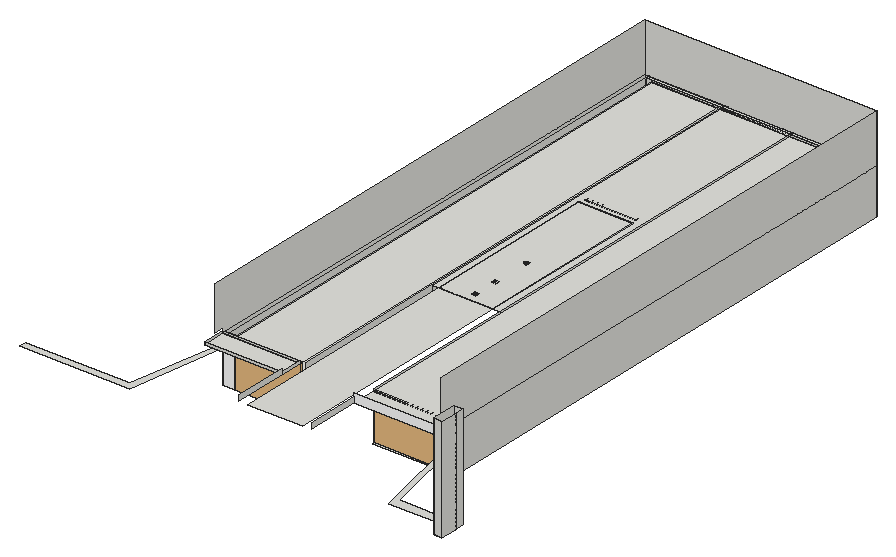
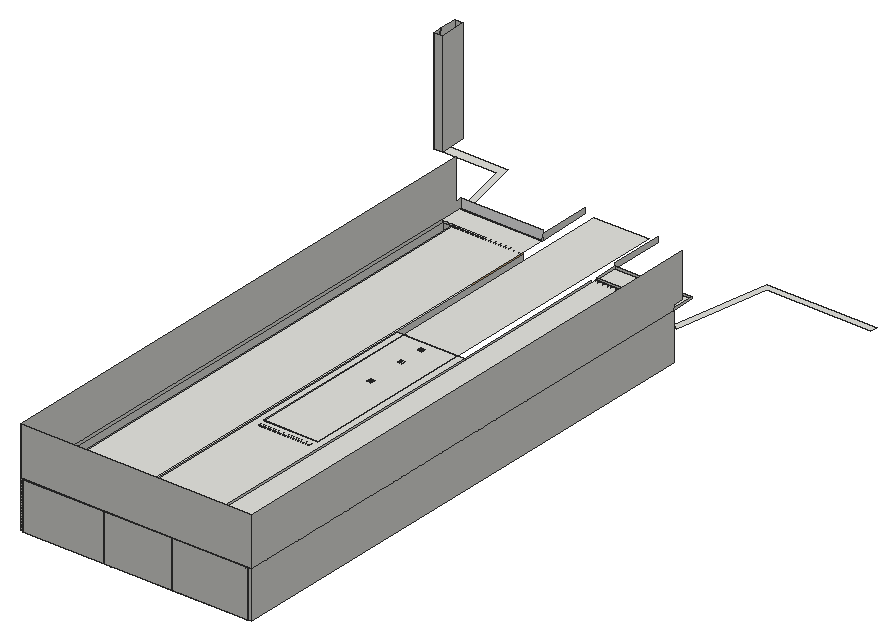
# SketchUp Ruby script. Lengths in inches.
U = 1.inch
M = Sketchup.active_model
def pt(a) = Geom::Point3d.new(a.map { |v| v * U })
def face(e, loops, mat)
  f = e.add_face(loops[0].map { |a| pt(a) })
  loops[1..].each { |l| e.add_face(l.map { |a| pt(a) }).erase! }
  f.material = f.back_material = mat if mat
  f
end
# faces: each face lists its corners as indices into pts; further lists are holes
def faces(e, pts, list, mat = nil) = list.each { |f| face(e, (f[0].is_a?(Array) ? f : [f]).map { |l| l.map { |i| pts[i] } }, mat) }
# xy, xz, yz: faces in a plane at the given z, y or x. An outline is a flat list of corners, or four numbers for a rectangle; further outlines are holes
def ring(l) = l.size == 4 ? [[l[0], l[1]], [l[2], l[1]], [l[2], l[3]], [l[0], l[3]]] : l.each_slice(2).to_a
def flat(e, list, mat, &to3) = list.each { |f| face(e, (f[0].is_a?(Array) ? f : [f]).map { |l| ring(l).map { |u, v| to3.(u, v) } }, mat) }
def xy(e, z, list, mat = nil) = flat(e, list, mat) { |x, y| [x, y, z] }
def xz(e, y, list, mat = nil) = flat(e, list, mat) { |x, z| [x, y, z] }
def yz(e, x, list, mat = nil) = flat(e, list, mat) { |y, z| [x, y, z] }
def lines(e, pts, list) = list.each { |a, b| e.add_line(pt(pts[a]), pt(pts[b])) }
# prism: a flat outline (further loops are holes) pulled along v
def prism(e, loops, v, mat = nil)
  f = face(e, loops, mat); d = Geom::Vector3d.new(v.map { |x| x * U })
  f.pushpull(f.normal.samedirection?(d) ? d.length : -d.length)
end
def box(e, o, s, mat = nil) = prism(e, [[o, [o[0] + s[0], o[1], o[2]], [o[0] + s[0], o[1] + s[1], o[2]], [o[0], o[1] + s[1], o[2]]]], [0, 0, s[2]], mat)
def at(x, y, z, deg = 0) = Geom::Transformation.translation(pt([x, y, z])) * Geom::Transformation.rotation(ORIGIN, Z_AXIS, deg.degrees)
def axes(o, x, y, z) = Geom::Transformation.new([*x, 0, *y, 0, *z, 0, *pt(o).to_a, 1])
def part(name) = M.definitions.add(name)
# library, detail: a bought-in or finely detailed component or shape, given as its bounding box
def library(name, o, s) = part(name).tap { |d| box(d.entities, o, s) }
def detail(e, o, s) = box(e.add_group.entities, o, s)
def put(e, d, t, mat = nil) = e.add_instance(d, t).tap { |i| i.material = mat if mat }
def group(e, t, mat = nil) = e.add_group.tap { |g| g.transformation = t; g.material = mat if mat }.entities
root = M.entities
M.materials.add("[Color M00]").color = [255, 255, 255]
c1 = library("Group\#4",[0,0,0],[146.0625,8.01,104.72])
c2 = library("Sliding Door",[0,0,0],[94.49,5.83,91.73])
c3 = library("Group5_1",[-7.56,-66.38,0.11],[6.33,135.04,120.95])
c4 = library("Omni Light\#4",[-12,-12,-12],[24,24,24])
c5 = library("Omni Light\#3",[-12,-12,-12],[24,24,24])
c6 = library("Spot Light",[-5.1,-5.1,-11.05],[10.2,10.2,11.05])
c7 = library("Spot Light\#1",[-5.1,-5.1,-11.05],[10.2,10.2,11.05])
c8 = library("Spot Light\#2",[-5.1,-5.1,-11.05],[10.2,10.2,11.05])
xy(root,34.97,[[765.09,749.51,934.66,2093.94],[1121.6,749.51,1301.45,2093.94],[744.92,758.51,765.09,758.51,765.09,2093.94,934.66,2093.94,934.66,976.22,940.98,976.22,940.98,2100.75,744.92,2100.75],[934.66,758.51,940.98,928.22],[1115.98,758.51,1121.6,758.51,1121.6,2093.94,1301.45,2093.94,1301.45,758.51,1323.45,758.51,1323.45,2100.75,1115.98,2100.75],
  [934.66,928.22,940.98,976.22],[940.98,2093.94,963.8,2100.75],[963.8,2093.94,1093.61,2100.75],[1093.61,2093.94,1115.98,2100.75],[744.92,2100.75,940.98,2109.75],
  [940.98,2100.75,963.8,2109.75],[963.8,2100.75,1093.61,2109.75],[1093.61,2100.75,1115.98,2109.75],[1115.98,2100.75,1323.45,2109.75],[744.92,2109.75,963.8,2111.5625],
  [963.8,2109.75,1093.61,2111.5625],[1093.61,2109.75,1323.45,2111.5625]])
xy(root,118.97,[[934.66,928.22,940.98,976.22],[940.98,928.22,958.48,976.22],[1098.48,937.55,1107.36,985.55]])
xy(root,120.65,[[1545.43,417,1548.46,459.625],[1548.46,417,1566.68,459.625],[1395.9,459.625,1545.43,459.625,1545.43,482.75,1404.4,482.75,1345.66,749.51,1332.45,749.51],[1545.43,459.625,1548.46,482.75],[1548.46,459.625,1566.68,463.0625],
  [1548.46,463.0625,1566.68,482.75],[411.47,500.87,693.04,500.87,735.92,749.51,721.7,754.86,678.72,519.18,411.47,519.18]])
xy(root,148.22,[[963.8,1617.7,1093.61,2109.75]])
xy(root,154.53,[[[958.48,1166.95,1098.48,1617.7],[1031.74,1351.9,1032.77,1352.04,1033.74,1352.4375,1034.57,1353.07,1035.2,1353.9,1035.6,1354.87,1035.74,1355.9,1035.6,1356.9375,1035.2,1357.9,1034.57,1358.73,1033.74,1359.37,1032.77,1359.76,1031.74,1359.9,1030.7,1359.76,1029.74,1359.37,1028.91,1358.73,1028.28,1357.9,1027.875,1356.9375,1027.74,1355.9,1027.875,1354.87,1028.28,1353.9,1028.91,1353.07,1029.74,1352.4375,1030.7,1352.04],[1031.74,1189.09,1032.77,1189.23,1033.74,1189.625,1034.57,1190.26,1035.2,1191.09,1035.6,1192.06,1035.74,1193.09,1035.6,1194.125,1035.2,1195.09,1034.57,1195.92,1033.74,1196.55,1032.77,1196.95,1031.74,1197.09,1030.7,1196.95,1029.74,1196.55,1028.91,1195.92,1028.28,1195.09,1027.875,1194.125,1027.74,1193.09,1027.875,1192.06,1028.28,1191.09,1028.91,1190.26,1029.74,1189.625,1030.7,1189.23],[1031.74,1254.99,1032.16,1255.05,1032.55,1255.21,1032.89,1255.47,1033.15,1255.81,1033.31,1256.2,1033.36,1256.62,1033.31,1257.04,1033.15,1257.43,1032.89,1257.77,1032.55,1258.03,1032.16,1258.1875,1031.74,1258.24,1031.32,1258.1875,1030.93,1258.03,1030.59,1257.77,1030.33,1257.43,1030.17,1257.04,1030.11,1256.62,1030.17,1256.2,1030.33,1255.81,1030.59,1255.47,1030.93,1255.21,1031.32,1255.05]]])
xy(root,154.97,[[958.48,552.07,1098.48,1166.95],[735.92,689.01,934.66,749.51],[1121.6,689.01,1332.45,692.91],[1121.6,692.91,1121.6,2093.94,1301.45,2093.94,1301.45,749.51,1332.45,749.51,1332.45,692.91],[765.09,749.51,934.66,2093.94],
  [940.98,1166.95,958.48,1166.95,958.48,1617.7,1098.48,1617.7,1098.48,1166.95,1115.98,1166.95,1115.98,2093.94,940.98,2093.94],[958.48,1166.95,1098.48,1617.7],[940.98,2093.94,1115.98,2100.75],[744.92,2100.75,940.98,2109.75],[940.98,2100.75,1115.98,2109.75],
  [1115.98,2100.75,1323.45,2109.75],[744.92,2109.75,1323.45,2111.5625]])
xy(root,155.84,[[1031.74,1189.09,1030.7,1189.23,1029.74,1189.625,1028.91,1190.26,1028.28,1191.09,1027.875,1192.06,1027.74,1193.09,1027.875,1194.125,1028.28,1195.09,1028.91,1195.92,1029.74,1196.55,1030.7,1196.95,1031.74,1197.09,1032.77,1196.95,1033.74,1196.55,1034.57,1195.92,1035.2,1195.09,1035.6,1194.125,1035.74,1193.09,1035.6,1192.06,1035.2,1191.09,1034.57,1190.26,1033.74,1189.625,1032.77,1189.23],[1031.74,1254.99,1031.32,1255.05,1030.93,1255.21,1030.59,1255.47,1030.33,1255.81,1030.17,1256.2,1030.11,1256.62,1030.17,1257.04,1030.33,1257.43,1030.59,1257.77,1030.93,1258.03,1031.32,1258.1875,1031.74,1258.24,1032.16,1258.1875,1032.55,1258.03,1032.89,1257.77,1033.15,1257.43,1033.31,1257.04,1033.36,1256.62,1033.31,1256.2,1033.15,1255.81,1032.89,1255.47,1032.55,1255.21,1032.16,1255.05],[1031.74,1351.9,1030.7,1352.04,1029.74,1352.4375,1028.91,1353.07,1028.28,1353.9,1027.875,1354.87,1027.74,1355.9,1027.875,1356.9375,1028.28,1357.9,1028.91,1358.73,1029.74,1359.37,1030.7,1359.76,1031.74,1359.9,1032.77,1359.76,1033.74,1359.37,1034.57,1358.73,1035.2,1357.9,1035.6,1356.9375,1035.74,1355.9,1035.6,1354.87,1035.2,1353.9,1034.57,1353.07,1033.74,1352.4375,1032.77,1352.04]])
xz(root,417,[[1545.43,120.65,1566.68,388.75]])
xz(root,482.75,[[1545.43,120.65,1566.68,388.75]])
xz(root,689.01,[[735.92,154.97,934.66,160.97]])
xz(root,689.01,[[1121.6,154.97,1332.45,178.15]],"[Color M00]")
xz(root,749.51,[[735.92,154.97,934.66,160.97]])
xz(root,749.51,[[735.92,34.97,765.09,154.97],[1301.45,34.97,1332.45,154.97]],"[Color M00]")
xz(root,758.51,[[744.92,34.97,765.09,154.97],[1301.45,34.97,1323.45,154.97]])
xz(root,928.22,[[934.66,34.97,940.98,118.97]])
xz(root,976.22,[[934.66,34.97,940.98,118.97]])
xz(root,1166.95,[[958.48,154.53,1098.48,154.97]])
xz(root,1617.7,[[958.48,154.53,1098.48,154.97]])
xz(root,2093.94,[[765.09,34.97,934.66,154.97],[940.98,34.97,1115.98,154.97],[1121.6,34.97,1301.45,154.97]])
xz(root,2100.75,[[744.92,34.97,1323.45,154.97]])
xz(root,2109.75,[[735.92,34.97,940.98,154.97],[940.98,34.97,940.98,154.97,1115.98,154.97,1115.98,34.97,1093.61,34.97,1093.61,148.22,963.8,148.22,963.8,34.97],[963.8,34.97,1093.61,148.22],[1115.98,34.97,1332.45,154.97],[735.92,154.97,1332.45,280.97]])
xz(root,2111.5625,[[744.92,34.97,1323.45,154.97]])
yz(root,735.92,[[749.51,34.97,2109.75,154.97],[689.01,154.97,749.51,160.97],[749.51,154.97,749.51,167.65,723.48,167.65,723.48,280.97,2109.75,280.97,2109.75,154.97]])
yz(root,744.92,[[758.51,34.97,2100.75,154.97],[2100.75,34.97,2111.5625,154.97]])
yz(root,765.09,[[749.51,34.97,758.51,154.97],[758.51,34.97,2093.94,154.97]])
yz(root,934.66,[[552.07,154.97,689.01,169.65],[689.01,154.97,749.51,160.97]])
yz(root,940.98,[[758.51,34.97,758.51,154.97,1166.95,154.97,1166.95,34.97,976.22,34.97,976.22,118.97,928.22,118.97,928.22,34.97],[1166.95,34.97,2093.94,154.97],[2093.94,34.97,2109.75,154.97]])
yz(root,958.48,[[1166.95,154.53,1617.7,154.97]])
yz(root,1098.48,[[1166.95,154.53,1617.7,154.97]])
yz(root,1115.98,[[758.51,34.97,1166.95,154.97],[1166.95,34.97,2093.94,154.97],[2093.94,34.97,2109.75,154.97]])
yz(root,1121.6,[[552.07,154.97,689.01,169.65],[689.01,154.97,692.91,160.97]])
yz(root,1301.45,[[749.51,34.97,758.51,154.97],[758.51,34.97,2093.94,154.97]])
yz(root,1323.45,[[758.51,34.97,2100.75,154.97],[2100.75,34.97,2111.5625,154.97]])
yz(root,1332.45,[[749.51,34.97,2109.75,154.97],[689.01,154.97,2109.75,154.97,2109.75,280.97,706.73,280.97,706.73,178.15,689.01,178.15]])
yz(root,1545.43,[[417,120.65,482.75,388.75]])
yz(root,1566.68,[[417,120.65,459.625,388.75],[459.625,120.65,463.0625,388.75],[463.0625,120.65,482.75,388.75]])
p = [[1031.74,1189.09,154.53],[1030.7,1189.23,154.53],[1030.7,1189.23,155.84],[1031.74,1189.09,155.84],[1032.77,1189.23,154.53],[1032.77,1189.23,155.84],
  [1029.74,1189.625,154.53],[1029.74,1189.625,155.84],[1033.74,1189.625,154.53],[1033.74,1189.625,155.84],[1028.91,1190.26,154.53],[1028.91,1190.26,155.84],
  [1034.57,1190.26,154.53],[1034.57,1190.26,155.84],[1028.28,1191.09,154.53],[1028.28,1191.09,155.84],[1035.2,1191.09,154.53],[1035.2,1191.09,155.84],
  [1027.875,1192.06,154.53],[1027.875,1192.06,155.84],[1035.6,1192.06,154.53],[1035.6,1192.06,155.84],[1027.74,1193.09,154.53],[1027.74,1193.09,155.84],
  [1035.74,1193.09,154.53],[1035.74,1193.09,155.84],[1027.875,1194.125,154.53],[1027.875,1194.125,155.84],[1035.6,1194.125,154.53],[1035.6,1194.125,155.84],
  [1028.28,1195.09,154.53],[1028.28,1195.09,155.84],[1035.2,1195.09,154.53],[1035.2,1195.09,155.84],[1028.91,1195.92,154.53],[1028.91,1195.92,155.84],
  [1034.57,1195.92,154.53],[1034.57,1195.92,155.84],[1029.74,1196.55,154.53],[1029.74,1196.55,155.84],[1033.74,1196.55,154.53],[1033.74,1196.55,155.84],
  [1030.7,1196.95,154.53],[1030.7,1196.95,155.84],[1032.77,1196.95,154.53],[1032.77,1196.95,155.84],[1031.74,1197.09,154.53],[1031.74,1197.09,155.84],
  [1031.32,1255.05,154.53],[1030.93,1255.21,154.53],[1030.93,1255.21,155.84],[1031.32,1255.05,155.84],[1031.74,1254.99,154.53],[1031.74,1254.99,155.84],
  [1032.16,1255.05,154.53],[1032.16,1255.05,155.84],[1032.55,1255.21,154.53],[1032.55,1255.21,155.84],[1030.59,1255.47,154.53],[1030.59,1255.47,155.84],
  [1032.89,1255.47,154.53],[1032.89,1255.47,155.84],[1030.33,1255.81,154.53],[1030.33,1255.81,155.84],[1033.15,1255.81,154.53],[1033.15,1255.81,155.84],
  [1030.17,1256.2,154.53],[1030.17,1256.2,155.84],[1033.31,1256.2,154.53],[1033.31,1256.2,155.84],[1030.11,1256.62,154.53],[1030.11,1256.62,155.84],
  [1033.36,1256.62,154.53],[1033.36,1256.62,155.84],[1030.17,1257.04,154.53],[1030.17,1257.04,155.84],[1033.31,1257.04,154.53],[1033.31,1257.04,155.84],
  [1030.33,1257.43,154.53],[1030.33,1257.43,155.84],[1033.15,1257.43,154.53],[1033.15,1257.43,155.84],[1030.59,1257.77,154.53],[1030.59,1257.77,155.84],
  [1032.89,1257.77,154.53],[1032.89,1257.77,155.84],[1030.93,1258.03,154.53],[1030.93,1258.03,155.84],[1032.55,1258.03,154.53],[1032.55,1258.03,155.84],
  [1031.32,1258.1875,154.53],[1031.32,1258.1875,155.84],[1032.16,1258.1875,154.53],[1032.16,1258.1875,155.84],[1031.74,1258.24,154.53],[1031.74,1258.24,155.84],
  [1031.74,1351.9,154.53],[1030.7,1352.04,154.53],[1030.7,1352.04,155.84],[1031.74,1351.9,155.84],[1032.77,1352.04,154.53],[1032.77,1352.04,155.84],
  [1029.74,1352.4375,154.53],[1029.74,1352.4375,155.84],[1033.74,1352.4375,154.53],[1033.74,1352.4375,155.84],[1028.91,1353.07,154.53],[1028.91,1353.07,155.84],
  [1034.57,1353.07,154.53],[1034.57,1353.07,155.84],[1028.28,1353.9,154.53],[1028.28,1353.9,155.84],[1035.2,1353.9,154.53],[1035.2,1353.9,155.84],
  [1027.875,1354.87,154.53],[1027.875,1354.87,155.84],[1035.6,1354.87,154.53],[1035.6,1354.87,155.84],[1027.74,1355.9,154.53],[1027.74,1355.9,155.84],
  [1035.74,1355.9,154.53],[1035.74,1355.9,155.84],[1027.875,1356.9375,154.53],[1027.875,1356.9375,155.84],[1035.6,1356.9375,154.53],[1035.6,1356.9375,155.84],
  [1028.28,1357.9,154.53],[1028.28,1357.9,155.84],[1035.2,1357.9,154.53],[1035.2,1357.9,155.84],[1028.91,1358.73,154.53],[1028.91,1358.73,155.84],
  [1034.57,1358.73,154.53],[1034.57,1358.73,155.84],[1029.74,1359.37,154.53],[1029.74,1359.37,155.84],[1033.74,1359.37,154.53],[1033.74,1359.37,155.84],
  [1030.7,1359.76,154.53],[1030.7,1359.76,155.84],[1032.77,1359.76,154.53],[1032.77,1359.76,155.84],[1031.74,1359.9,154.53],[1031.74,1359.9,155.84],
  [1115.98,758.51,154.97],[1121.6,758.51,154.97],[934.66,758.51,154.97],[940.98,758.51,154.97]]
faces(root,p,[[0,1,2,3],[4,0,3,5],[1,6,7,2],[8,4,5,9],[6,10,11,7],[12,8,9,13],[10,14,15,11],[16,12,13,17],
  [14,18,19,15],[20,16,17,21],[18,22,23,19],[24,20,21,25],[22,26,27,23],[28,24,25,29],[26,30,31,27],[32,28,29,33],
  [30,34,35,31],[36,32,33,37],[34,38,39,35],[40,36,37,41],[38,42,43,39],[44,40,41,45],[42,46,47,43],[46,44,45,47],
  [48,49,50,51],[52,48,51,53],[54,52,53,55],[56,54,55,57],[49,58,59,50],[60,56,57,61],[58,62,63,59],[64,60,61,65],
  [62,66,67,63],[68,64,65,69],[66,70,71,67],[72,68,69,73],[70,74,75,71],[76,72,73,77],[74,78,79,75],[80,76,77,81],
  [78,82,83,79],[84,80,81,85],[82,86,87,83],[88,84,85,89],[86,90,91,87],[92,88,89,93],[90,94,95,91],[94,92,93,95],
  [96,97,98,99],[100,96,99,101],[97,102,103,98],[104,100,101,105],[102,106,107,103],[108,104,105,109],[106,110,111,107],[112,108,109,113],
  [110,114,115,111],[116,112,113,117],[114,118,119,115],[120,116,117,121],[118,122,123,119],[124,120,121,125],[122,126,127,123],[128,124,125,129],
  [126,130,131,127],[132,128,129,133],[130,134,135,131],[136,132,133,137],[134,138,139,135],[140,136,137,141],[138,142,143,139],[142,140,141,143]])
lines(root,p,[[144,145],[146,147]])
put(root,c1,axes([963.8,1632.01,34.97],[0.88874,0,0],[0,1,0],[0,0,1.14586]))
put(root,c2,axes([765.09,749.51,34.97],[1.79644,0,0],[0,1,0],[0,0,1.30815]))
put(root,c3,axes([1210.01,750.95,37.54],[0,-1,0],[1.33185,0,0],[0,0,0.97]))
put(root,c4,axes([1035.48,1602,89.64],[2,0,0],[0,2,0],[0,0,2]))
put(root,c5,at(1032.12,1198.34,138.81))
put(root,c5,at(1032.12,1332.28,138.81))
put(root,c6,at(1031.74,1193.09,154.52))
put(root,c7,at(1031.74,1256.62,154.52))
put(root,c8,at(1031.74,1355.65,154.52))
